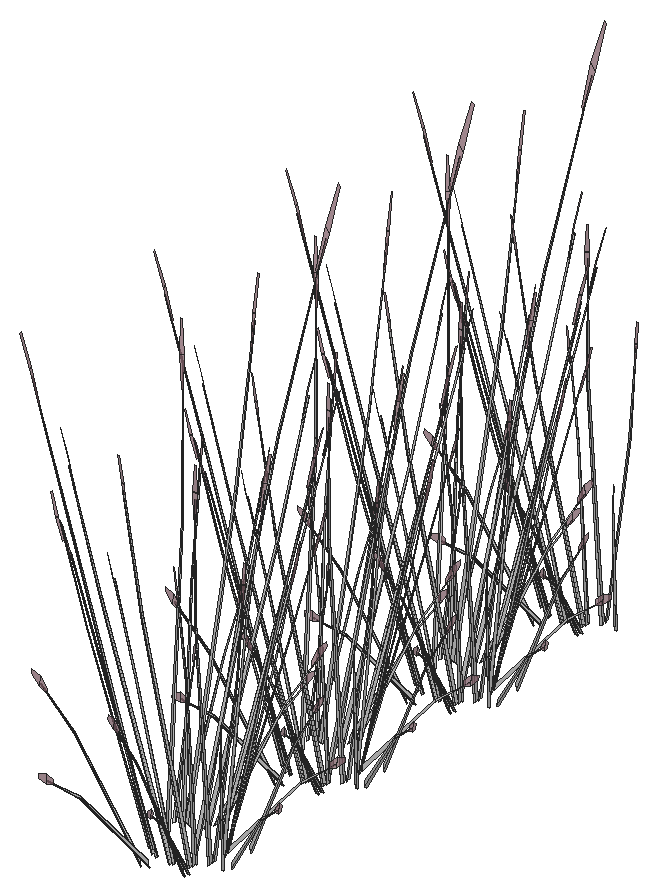
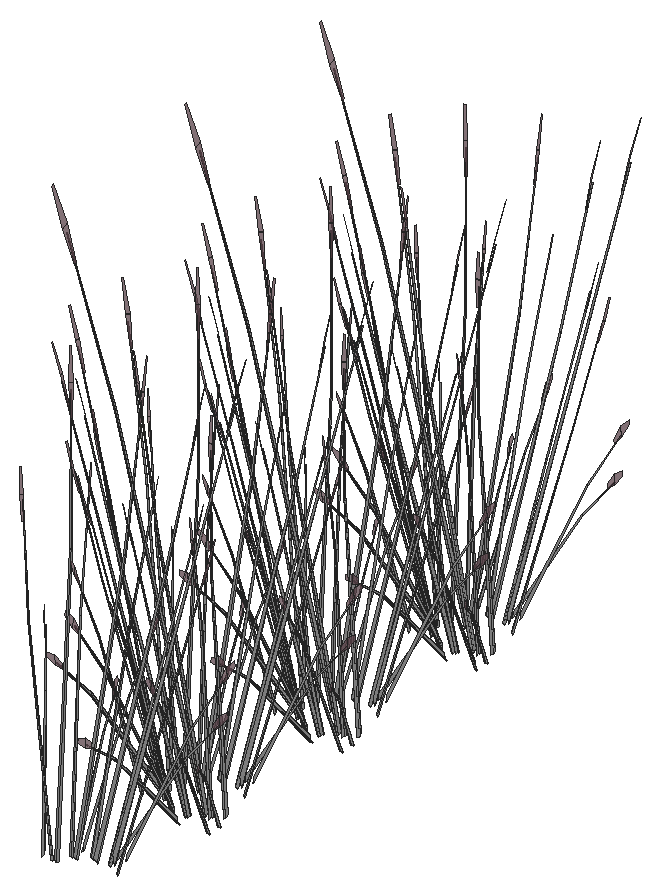
# SketchUp Ruby script. Lengths in inches.
U = 1.inch
M = Sketchup.active_model
def pt(a) = Geom::Point3d.new(a.map { |v| v * U })
def face(e, loops, mat)
  f = e.add_face(loops[0].map { |a| pt(a) })
  loops[1..].each { |l| e.add_face(l.map { |a| pt(a) }).erase! }
  f.material = f.back_material = mat if mat
  f
end
# faces: each face lists its corners as indices into pts; further lists are holes
def faces(e, pts, list, mat = nil) = list.each { |f| face(e, (f[0].is_a?(Array) ? f : [f]).map { |l| l.map { |i| pts[i] } }, mat) }
# xy, xz, yz: faces in a plane at the given z, y or x. An outline is a flat list of corners, or four numbers for a rectangle; further outlines are holes
def ring(l) = l.size == 4 ? [[l[0], l[1]], [l[2], l[1]], [l[2], l[3]], [l[0], l[3]]] : l.each_slice(2).to_a
def flat(e, list, mat, &to3) = list.each { |f| face(e, (f[0].is_a?(Array) ? f : [f]).map { |l| ring(l).map { |u, v| to3.(u, v) } }, mat) }
def xy(e, z, list, mat = nil) = flat(e, list, mat) { |x, y| [x, y, z] }
def xz(e, y, list, mat = nil) = flat(e, list, mat) { |x, z| [x, y, z] }
def yz(e, x, list, mat = nil) = flat(e, list, mat) { |y, z| [x, y, z] }
def lines(e, pts, list) = list.each { |a, b| e.add_line(pt(pts[a]), pt(pts[b])) }
# prism: a flat outline (further loops are holes) pulled along v
def prism(e, loops, v, mat = nil)
  f = face(e, loops, mat); d = Geom::Vector3d.new(v.map { |x| x * U })
  f.pushpull(f.normal.samedirection?(d) ? d.length : -d.length)
end
def box(e, o, s, mat = nil) = prism(e, [[o, [o[0] + s[0], o[1], o[2]], [o[0] + s[0], o[1] + s[1], o[2]], [o[0], o[1] + s[1], o[2]]]], [0, 0, s[2]], mat)
def at(x, y, z, deg = 0) = Geom::Transformation.translation(pt([x, y, z])) * Geom::Transformation.rotation(ORIGIN, Z_AXIS, deg.degrees)
def axes(o, x, y, z) = Geom::Transformation.new([*x, 0, *y, 0, *z, 0, *pt(o).to_a, 1])
def part(name) = M.definitions.add(name)
# library, detail: a bought-in or finely detailed component or shape, given as its bounding box
def library(name, o, s) = part(name).tap { |d| box(d.entities, o, s) }
def detail(e, o, s) = box(e.add_group.entities, o, s)
def put(e, d, t, mat = nil) = e.add_instance(d, t).tap { |i| i.material = mat if mat }
def group(e, t, mat = nil) = e.add_group.tap { |g| g.transformation = t; g.material = mat if mat }.entities
root = M.entities
M.materials.add("LightPink_Translucent").color = [144, 107, 117]
M.materials["LightPink_Translucent"].alpha = 0.75
M.materials.add("[_0053_Ivory_]").color = [200, 200, 200]
c1 = part("blade")
p = [[2.15,0.21,22],[0,0.17,0],[0.09,0.45,0],[2.18,0.31,22],[2.29,0.31,22],[0.38,0.45,0],
  [2.48,0.24,33],[2.49,0.24,33],[2.48,0.22,33]]
faces(c1.entities,p,[[0,1,2,3],[4,5,2,3],[6,3,4,7],[8,0,3,6]])
c2 = part("seeds")
p = [[0.3,-0.1,1.38],[-0.01,-0.03,1.59],[-0.01,-0.03,0.03],[0.14,-0.07,-0.07],[0.29,-0.03,3],[0.15,0.01,3.11]]
faces(c2.entities,p,[[0,1,2,3],[1,0,4,5]],"LightPink_Translucent")
c3 = part("blade with seeds")
put(c3.entities,c1,at(0,0,0))
put(c3.entities,c2,axes([2.4,0.25,30.99],[1.5799,-0.05474,1.17369],[-0.12525,1.92788,0.29478],[-0.07173,-0.02425,1.56792]))
put(root,c3,axes([643.55,105.5625,131.37],[-0.0929,-0.08817,1.74944],[-0.61994,0.0559,-0.27667],[-0.09894,-0.21089,0.14031]),"[_0053_Ivory_]")
put(root,c3,axes([646.33,106.64,131.37],[-0.00586,-0.12516,1.74944],[-0.49517,-0.36172,-0.27667],[0.07656,-0.21927,0.14031]),"[_0053_Ivory_]")
put(root,c3,axes([646.2,106.19,131.36],[-0.06168,0.04803,1.77383],[-0.60432,-0.16205,-0.16761],[-0.02188,-0.20961,0.31391]),"[_0053_Ivory_]")
put(root,c3,axes([642.91,105.27,131.36],[-0.01133,0.07538,1.77383],[-0.55883,0.27355,-0.16761],[-0.16445,-0.13983,0.31391]),"[_0053_Ivory_]")
put(root,c3,axes([644.49,106.92,131.6875],[-0.59433,0.29278,-0.1216],[-0.29207,-0.51964,-0.67495],[-0.07842,-0.21898,1.02557]),"[_0053_Ivory_]")
put(root,c3,axes([645.72,107.58,131.6875],[-0.6675,-0.03116,-0.1216],[0.01824,-0.58993,-0.67495],[0.04637,-0.2272,1.02557]),"[_0053_Ivory_]")
put(root,c3,axes([644.48,106.6875,131.38],[0.44753,-0.21372,0.0643],[0.21905,0.38973,0.50621],[-0.04322,-0.1718,0.77189]),"[_0053_Ivory_]")
put(root,c3,axes([642.94,106.75,131.38],[0.27604,-0.39948,0.0643],[0.39309,0.23258,0.50621],[-0.12709,-0.12808,0.77189]),"[_0053_Ivory_]")
put(root,c3,axes([643.07,106.71,132.08],[-0.40534,0.60286,-0.13619],[-0.58702,-0.34732,-0.75594],[-0.20405,-0.17032,1.14864]),"[_0053_Ivory_]")
put(root,c3,axes([645.84,107.37,131.38],[0.49911,0.0293,0.0643],[-0.01368,0.44245,0.50621],[0.05223,-0.16948,0.77189]),"[_0053_Ivory_]")
put(root,c3,axes([646.45,108.74,131.6875],[-0.56181,-0.34675,-0.1216],[0.32367,-0.50216,-0.67495],[0.15873,-0.17455,1.02557]),"[_0053_Ivory_]")
put(root,c3,axes([647.83,108.59,131.36],[-0.07933,-0.00478,1.77383],[-0.32942,-0.51175,-0.16761],[0.13229,-0.16826,0.31391]),"[_0053_Ivory_]")
put(root,c3,axes([641.65,107.53,131.38],[0.03058,-0.47819,0.0643],[0.4618,0.01311,0.50621],[-0.1769,-0.05004,0.77189]),"[_0053_Ivory_]")
put(root,c3,axes([646.66,108.61,131.38],[0.41695,0.26447,0.0643],[-0.24275,0.37662,0.50621],[0.13368,-0.12176,0.77189]),"[_0053_Ivory_]")
put(root,c3,axes([648.13,109.2,131.37],[0.08428,-0.09579,1.74944],[-0.10787,-0.58756,-0.27667],[0.21147,-0.1114,0.14031]),"[_0053_Ivory_]")
put(root,c3,axes([646.47,110.09,131.6875],[-0.30559,-0.56943,-0.1216],[0.54237,-0.27983,-0.67495],[0.22856,-0.07513,1.02557]),"[_0053_Ivory_]")
put(root,c3,axes([646.72,110.08,131.38],[0.22307,0.42878,0.0643],[-0.40677,0.20987,0.50621],[0.17931,-0.04141,0.77189]),"[_0053_Ivory_]")
put(root,c3,axes([647.6875,111.79,131.36],[-0.05492,-0.05505,1.77383],[0.12013,-0.59013,-0.16761],[0.21632,-0.0377,0.31391]),"[_0053_Ivory_]")
put(root,c3,axes([645.79,111.28,131.6875],[0.03252,-0.63953,-0.1216],[0.61574,0.01748,-0.67495],[0.23714,0.04442,1.02557]),"[_0053_Ivory_]")
put(root,c3,axes([646.32,110.89,131.37],[0.13029,-0.01064,1.74944],[0.35737,-0.48855,-0.27667],[0.23175,0.06449,0.14031]),"[_0053_Ivory_]")
put(root,c3,axes([646.01,111.38,131.38],[-0.03058,0.47819,0.0643],[-0.4618,-0.01311,0.50621],[0.1769,0.05004,0.77189]),"[_0053_Ivory_]")
put(root,c3,axes([644.98,108.8,131.13],[-0.52482,-0.32674,1.38283],[0.55416,-0.50872,0.59665],[0.16933,0.30658,1.33663]),"[_0053_Ivory_]")
put(root,c3,axes([641.2,110.18,131.6875],[0.56181,0.34675,-0.1216],[-0.32367,0.50216,-0.67495],[-0.15873,0.17455,1.02557]),"[_0053_Ivory_]")
put(root,c3,axes([644.57,111.97,131.6875],[0.36191,-0.53827,-0.1216],[0.52412,0.3101,-0.67495],[0.18219,0.15207,1.02557]),"[_0053_Ivory_]")
put(root,c3,axes([644.1,112.42,131.36],[0.0018,-0.07613,1.77383],[0.52048,-0.3359,-0.16761],[0.18079,0.11989,0.31391]),"[_0053_Ivory_]")
put(root,c3,axes([641.82,111.55,131.38],[-0.49911,-0.0293,0.0643],[0.01368,-0.44245,0.50621],[-0.05223,0.16948,0.77189]),"[_0053_Ivory_]")
put(root,c3,axes([644.71,112.17,131.38],[-0.27604,0.39948,0.0643],[-0.39309,-0.23258,0.50621],[0.12709,0.12808,0.77189]),"[_0053_Ivory_]")
put(root,c3,axes([643.18,112.23,131.38],[-0.44753,0.21372,0.0643],[-0.21905,-0.38973,0.50621],[0.04322,0.1718,0.77189]),"[_0053_Ivory_]")
put(root,c3,axes([640.56,111.62,131.37],[-0.0151,0.12444,1.74944],[0.42844,0.43292,-0.27667],[-0.11216,0.20472,0.14031]),"[_0053_Ivory_]")
put(root,c3,axes([641.93,111.34,132.05],[0.6675,0.03116,-0.13498],[-0.01824,0.58993,-0.74919],[-0.04637,0.2272,1.13838]),"[_0053_Ivory_]")
put(root,c3,axes([643.16,111.99,131.6875],[0.59433,-0.29278,-0.1216],[0.29207,0.51964,-0.67495],[0.07842,0.21898,1.02557]),"[_0053_Ivory_]")
put(root,c3,axes([643.55,120.625,131.37],[-0.0929,-0.08817,1.74944],[-0.61994,0.0559,-0.27667],[-0.09894,-0.21089,0.14031]),"[_0053_Ivory_]")
put(root,c3,axes([640.51,112.89,131.36],[0.0689,-0.03797,1.77383],[0.5695,0.25254,-0.16761],[-0.01338,0.21027,0.31391]),"[_0053_Ivory_]")
put(root,c3,axes([643.02,113.16,131.37],[0.07699,0.10127,1.74944],[0.6213,0.03978,-0.27667],[0.06248,0.22333,0.14031]),"[_0053_Ivory_]")
put(root,c3,axes([646.33,121.71,131.37],[-0.00586,-0.12516,1.74944],[-0.49517,-0.36172,-0.27667],[0.07656,-0.21927,0.14031]),"[_0053_Ivory_]")
put(root,c3,axes([646.2,121.26,131.36],[-0.06168,0.04803,1.77383],[-0.60432,-0.16205,-0.16761],[-0.02188,-0.20961,0.31391]),"[_0053_Ivory_]")
put(root,c3,axes([642.91,120.34,131.36],[-0.01133,0.07538,1.77383],[-0.55883,0.27355,-0.16761],[-0.16445,-0.13983,0.31391]),"[_0053_Ivory_]")
put(root,c3,axes([644.49,121.99,131.6875],[-0.59433,0.29278,-0.1216],[-0.29207,-0.51964,-0.67495],[-0.07842,-0.21898,1.02557]),"[_0053_Ivory_]")
put(root,c3,axes([645.72,122.64,131.6875],[-0.6675,-0.03116,-0.1216],[0.01824,-0.58993,-0.67495],[0.04637,-0.2272,1.02557]),"[_0053_Ivory_]")
put(root,c3,axes([644.48,121.75,131.38],[0.44753,-0.21372,0.0643],[0.21905,0.38973,0.50621],[-0.04322,-0.1718,0.77189]),"[_0053_Ivory_]")
put(root,c3,axes([642.94,121.8125,131.38],[0.27604,-0.39948,0.0643],[0.39309,0.23258,0.50621],[-0.12709,-0.12808,0.77189]),"[_0053_Ivory_]")
put(root,c3,axes([643.07,121.77,132.08],[-0.40534,0.60286,-0.13619],[-0.58702,-0.34732,-0.75594],[-0.20405,-0.17032,1.14864]),"[_0053_Ivory_]")
put(root,c3,axes([645.84,122.43,131.38],[0.49911,0.0293,0.0643],[-0.01368,0.44245,0.50621],[0.05223,-0.16948,0.77189]),"[_0053_Ivory_]")
put(root,c3,axes([646.45,123.81,131.6875],[-0.56181,-0.34675,-0.1216],[0.32367,-0.50216,-0.67495],[0.15873,-0.17455,1.02557]),"[_0053_Ivory_]")
put(root,c3,axes([647.83,123.65,131.36],[-0.07933,-0.00478,1.77383],[-0.32942,-0.51175,-0.16761],[0.13229,-0.16826,0.31391]),"[_0053_Ivory_]")
put(root,c3,axes([641.65,122.6,131.38],[0.03058,-0.47819,0.0643],[0.4618,0.01311,0.50621],[-0.1769,-0.05004,0.77189]),"[_0053_Ivory_]")
put(root,c3,axes([646.66,123.68,131.38],[0.41695,0.26447,0.0643],[-0.24275,0.37662,0.50621],[0.13368,-0.12176,0.77189]),"[_0053_Ivory_]")
put(root,c3,axes([648.13,124.27,131.37],[0.08428,-0.09579,1.74944],[-0.10787,-0.58756,-0.27667],[0.21147,-0.1114,0.14031]),"[_0053_Ivory_]")
put(root,c3,axes([646.47,125.16,131.6875],[-0.30559,-0.56943,-0.1216],[0.54237,-0.27983,-0.67495],[0.22856,-0.07513,1.02557]),"[_0053_Ivory_]")
put(root,c3,axes([646.72,125.15,131.38],[0.22307,0.42878,0.0643],[-0.40677,0.20987,0.50621],[0.17931,-0.04141,0.77189]),"[_0053_Ivory_]")
put(root,c3,axes([647.6875,126.85,131.36],[-0.05492,-0.05505,1.77383],[0.12013,-0.59013,-0.16761],[0.21632,-0.0377,0.31391]),"[_0053_Ivory_]")
put(root,c3,axes([645.79,126.34,131.6875],[0.03252,-0.63953,-0.1216],[0.61574,0.01748,-0.67495],[0.23714,0.04442,1.02557]),"[_0053_Ivory_]")
put(root,c3,axes([646.32,125.96,131.37],[0.13029,-0.01064,1.74944],[0.35737,-0.48855,-0.27667],[0.23175,0.06449,0.14031]),"[_0053_Ivory_]")
put(root,c3,axes([646.01,126.45,131.38],[-0.03058,0.47819,0.0643],[-0.4618,-0.01311,0.50621],[0.1769,0.05004,0.77189]),"[_0053_Ivory_]")
put(root,c3,axes([644.98,123.86,131.13],[-0.52482,-0.32674,1.38283],[0.55416,-0.50872,0.59665],[0.16933,0.30658,1.33663]),"[_0053_Ivory_]")
put(root,c3,axes([641.2,125.24,131.6875],[0.56181,0.34675,-0.1216],[-0.32367,0.50216,-0.67495],[-0.15873,0.17455,1.02557]),"[_0053_Ivory_]")
put(root,c3,axes([644.57,127.04,131.6875],[0.36191,-0.53827,-0.1216],[0.52412,0.3101,-0.67495],[0.18219,0.15207,1.02557]),"[_0053_Ivory_]")
put(root,c3,axes([644.1,127.48,131.36],[0.0018,-0.07613,1.77383],[0.52048,-0.3359,-0.16761],[0.18079,0.11989,0.31391]),"[_0053_Ivory_]")
put(root,c3,axes([641.82,126.61,131.38],[-0.49911,-0.0293,0.0643],[0.01368,-0.44245,0.50621],[-0.05223,0.16948,0.77189]),"[_0053_Ivory_]")
put(root,c3,axes([644.71,127.23,131.38],[-0.27604,0.39948,0.0643],[-0.39309,-0.23258,0.50621],[0.12709,0.12808,0.77189]),"[_0053_Ivory_]")
put(root,c3,axes([643.18,127.29,131.38],[-0.44753,0.21372,0.0643],[-0.21905,-0.38973,0.50621],[0.04322,0.1718,0.77189]),"[_0053_Ivory_]")
put(root,c3,axes([640.56,126.68,131.37],[-0.0151,0.12444,1.74944],[0.42844,0.43292,-0.27667],[-0.11216,0.20472,0.14031]),"[_0053_Ivory_]")
put(root,c3,axes([641.93,126.4,132.05],[0.6675,0.03116,-0.13498],[-0.01824,0.58993,-0.74919],[-0.04637,0.2272,1.13838]),"[_0053_Ivory_]")
put(root,c3,axes([643.16,127.06,131.6875],[0.59433,-0.29278,-0.1216],[0.29207,0.51964,-0.67495],[0.07842,0.21898,1.02557]),"[_0053_Ivory_]")
put(root,c3,axes([643.55,135.54,131.37],[-0.0929,-0.08817,1.74944],[-0.61994,0.0559,-0.27667],[-0.09894,-0.21089,0.14031]),"[_0053_Ivory_]")
put(root,c3,axes([640.51,127.96,131.36],[0.0689,-0.03797,1.77383],[0.5695,0.25254,-0.16761],[-0.01338,0.21027,0.31391]),"[_0053_Ivory_]")
put(root,c3,axes([646.33,136.62,131.37],[-0.00586,-0.12516,1.74944],[-0.49517,-0.36172,-0.27667],[0.07656,-0.21927,0.14031]),"[_0053_Ivory_]")
put(root,c3,axes([646.2,136.17,131.36],[-0.06168,0.04803,1.77383],[-0.60432,-0.16205,-0.16761],[-0.02188,-0.20961,0.31391]),"[_0053_Ivory_]")
put(root,c3,axes([643.02,128.22,131.37],[0.07699,0.10127,1.74944],[0.6213,0.03978,-0.27667],[0.06248,0.22333,0.14031]),"[_0053_Ivory_]")
put(root,c3,axes([642.91,135.25,131.36],[-0.01133,0.07538,1.77383],[-0.55883,0.27355,-0.16761],[-0.16445,-0.13983,0.31391]),"[_0053_Ivory_]")
put(root,c3,axes([644.49,136.9,131.6875],[-0.59433,0.29278,-0.1216],[-0.29207,-0.51964,-0.67495],[-0.07842,-0.21898,1.02557]),"[_0053_Ivory_]")
put(root,c3,axes([645.72,137.56,131.6875],[-0.6675,-0.03116,-0.1216],[0.01824,-0.58993,-0.67495],[0.04637,-0.2272,1.02557]),"[_0053_Ivory_]")
put(root,c3,axes([644.48,136.67,131.38],[0.44753,-0.21372,0.0643],[0.21905,0.38973,0.50621],[-0.04322,-0.1718,0.77189]),"[_0053_Ivory_]")
put(root,c3,axes([642.94,136.73,131.38],[0.27604,-0.39948,0.0643],[0.39309,0.23258,0.50621],[-0.12709,-0.12808,0.77189]),"[_0053_Ivory_]")
put(root,c3,axes([643.07,136.69,132.08],[-0.40534,0.60286,-0.13619],[-0.58702,-0.34732,-0.75594],[-0.20405,-0.17032,1.14864]),"[_0053_Ivory_]")
put(root,c3,axes([645.84,137.35,131.38],[0.49911,0.0293,0.0643],[-0.01368,0.44245,0.50621],[0.05223,-0.16948,0.77189]),"[_0053_Ivory_]")
put(root,c3,axes([646.45,138.72,131.6875],[-0.56181,-0.34675,-0.1216],[0.32367,-0.50216,-0.67495],[0.15873,-0.17455,1.02557]),"[_0053_Ivory_]")
put(root,c3,axes([647.83,138.57,131.36],[-0.07933,-0.00478,1.77383],[-0.32942,-0.51175,-0.16761],[0.13229,-0.16826,0.31391]),"[_0053_Ivory_]")
put(root,c3,axes([641.65,137.51,131.38],[0.03058,-0.47819,0.0643],[0.4618,0.01311,0.50621],[-0.1769,-0.05004,0.77189]),"[_0053_Ivory_]")
put(root,c3,axes([646.66,138.59,131.38],[0.41695,0.26447,0.0643],[-0.24275,0.37662,0.50621],[0.13368,-0.12176,0.77189]),"[_0053_Ivory_]")
put(root,c3,axes([648.13,139.18,131.37],[0.08428,-0.09579,1.74944],[-0.10787,-0.58756,-0.27667],[0.21147,-0.1114,0.14031]),"[_0053_Ivory_]")
put(root,c3,axes([646.47,140.07,131.6875],[-0.30559,-0.56943,-0.1216],[0.54237,-0.27983,-0.67495],[0.22856,-0.07513,1.02557]),"[_0053_Ivory_]")
put(root,c3,axes([646.72,140.0625,131.38],[0.22307,0.42878,0.0643],[-0.40677,0.20987,0.50621],[0.17931,-0.04141,0.77189]),"[_0053_Ivory_]")
put(root,c3,axes([647.6875,141.77,131.36],[-0.05492,-0.05505,1.77383],[0.12013,-0.59013,-0.16761],[0.21632,-0.0377,0.31391]),"[_0053_Ivory_]")
put(root,c3,axes([645.79,141.26,131.6875],[0.03252,-0.63953,-0.1216],[0.61574,0.01748,-0.67495],[0.23714,0.04442,1.02557]),"[_0053_Ivory_]")
put(root,c3,axes([646.32,140.875,131.37],[0.13029,-0.01064,1.74944],[0.35737,-0.48855,-0.27667],[0.23175,0.06449,0.14031]),"[_0053_Ivory_]")
put(root,c3,axes([646.01,141.36,131.38],[-0.03058,0.47819,0.0643],[-0.4618,-0.01311,0.50621],[0.1769,0.05004,0.77189]),"[_0053_Ivory_]")
put(root,c3,axes([644.98,138.78,131.13],[-0.52482,-0.32674,1.38283],[0.55416,-0.50872,0.59665],[0.16933,0.30658,1.33663]),"[_0053_Ivory_]")
put(root,c3,axes([641.2,140.16,131.6875],[0.56181,0.34675,-0.1216],[-0.32367,0.50216,-0.67495],[-0.15873,0.17455,1.02557]),"[_0053_Ivory_]")
put(root,c3,axes([644.57,141.95,131.6875],[0.36191,-0.53827,-0.1216],[0.52412,0.3101,-0.67495],[0.18219,0.15207,1.02557]),"[_0053_Ivory_]")
put(root,c3,axes([644.1,142.4,131.36],[0.0018,-0.07613,1.77383],[0.52048,-0.3359,-0.16761],[0.18079,0.11989,0.31391]),"[_0053_Ivory_]")
put(root,c3,axes([641.82,141.53,131.38],[-0.49911,-0.0293,0.0643],[0.01368,-0.44245,0.50621],[-0.05223,0.16948,0.77189]),"[_0053_Ivory_]")
put(root,c3,axes([644.71,142.15,131.38],[-0.27604,0.39948,0.0643],[-0.39309,-0.23258,0.50621],[0.12709,0.12808,0.77189]),"[_0053_Ivory_]")
put(root,c3,axes([643.18,142.21,131.38],[-0.44753,0.21372,0.0643],[-0.21905,-0.38973,0.50621],[0.04322,0.1718,0.77189]),"[_0053_Ivory_]")
put(root,c3,axes([640.56,141.6,131.37],[-0.0151,0.12444,1.74944],[0.42844,0.43292,-0.27667],[-0.11216,0.20472,0.14031]),"[_0053_Ivory_]")
put(root,c3,axes([641.93,141.32,132.05],[0.6675,0.03116,-0.13498],[-0.01824,0.58993,-0.74919],[-0.04637,0.2272,1.13838]),"[_0053_Ivory_]")
put(root,c3,axes([643.16,141.97,131.6875],[0.59433,-0.29278,-0.1216],[0.29207,0.51964,-0.67495],[0.07842,0.21898,1.02557]),"[_0053_Ivory_]")
put(root,c3,axes([643.55,149.82,131.37],[-0.0929,-0.08817,1.74944],[-0.61994,0.0559,-0.27667],[-0.09894,-0.21089,0.14031]),"[_0053_Ivory_]")
put(root,c3,axes([646.33,150.9,131.37],[-0.00586,-0.12516,1.74944],[-0.49517,-0.36172,-0.27667],[0.07656,-0.21927,0.14031]),"[_0053_Ivory_]")
put(root,c3,axes([640.51,142.875,131.36],[0.0689,-0.03797,1.77383],[0.5695,0.25254,-0.16761],[-0.01338,0.21027,0.31391]),"[_0053_Ivory_]")
put(root,c3,axes([646.2,150.45,131.36],[-0.06168,0.04803,1.77383],[-0.60432,-0.16205,-0.16761],[-0.02188,-0.20961,0.31391]),"[_0053_Ivory_]")
put(root,c3,axes([642.91,149.53,131.36],[-0.01133,0.07538,1.77383],[-0.55883,0.27355,-0.16761],[-0.16445,-0.13983,0.31391]),"[_0053_Ivory_]")
put(root,c3,axes([643.02,143.14,131.37],[0.07699,0.10127,1.74944],[0.6213,0.03978,-0.27667],[0.06248,0.22333,0.14031]),"[_0053_Ivory_]")
put(root,c3,axes([644.49,151.18,131.6875],[-0.59433,0.29278,-0.1216],[-0.29207,-0.51964,-0.67495],[-0.07842,-0.21898,1.02557]),"[_0053_Ivory_]")
put(root,c3,axes([645.72,151.84,131.6875],[-0.6675,-0.03116,-0.1216],[0.01824,-0.58993,-0.67495],[0.04637,-0.2272,1.02557]),"[_0053_Ivory_]")
put(root,c3,axes([644.48,150.94,131.38],[0.44753,-0.21372,0.0643],[0.21905,0.38973,0.50621],[-0.04322,-0.1718,0.77189]),"[_0053_Ivory_]")
put(root,c3,axes([642.94,151,131.38],[0.27604,-0.39948,0.0643],[0.39309,0.23258,0.50621],[-0.12709,-0.12808,0.77189]),"[_0053_Ivory_]")
put(root,c3,axes([643.07,150.96,132.08],[-0.40534,0.60286,-0.13619],[-0.58702,-0.34732,-0.75594],[-0.20405,-0.17032,1.14864]),"[_0053_Ivory_]")
put(root,c3,axes([645.84,151.625,131.38],[0.49911,0.0293,0.0643],[-0.01368,0.44245,0.50621],[0.05223,-0.16948,0.77189]),"[_0053_Ivory_]")
put(root,c3,axes([646.45,153,131.6875],[-0.56181,-0.34675,-0.1216],[0.32367,-0.50216,-0.67495],[0.15873,-0.17455,1.02557]),"[_0053_Ivory_]")
put(root,c3,axes([647.83,152.85,131.36],[-0.07933,-0.00478,1.77383],[-0.32942,-0.51175,-0.16761],[0.13229,-0.16826,0.31391]),"[_0053_Ivory_]")
put(root,c3,axes([641.65,151.79,131.38],[0.03058,-0.47819,0.0643],[0.4618,0.01311,0.50621],[-0.1769,-0.05004,0.77189]),"[_0053_Ivory_]")
put(root,c3,axes([646.66,152.87,131.38],[0.41695,0.26447,0.0643],[-0.24275,0.37662,0.50621],[0.13368,-0.12176,0.77189]),"[_0053_Ivory_]")
